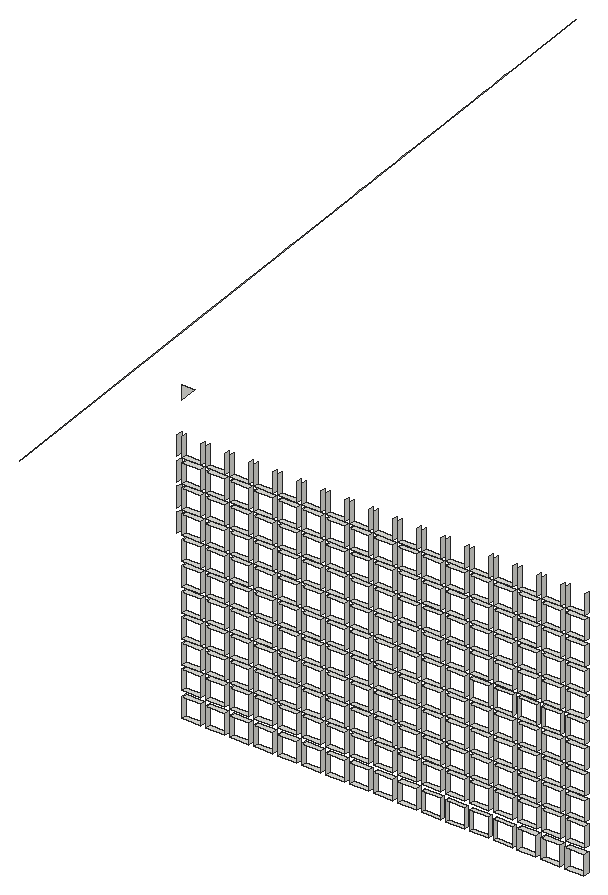
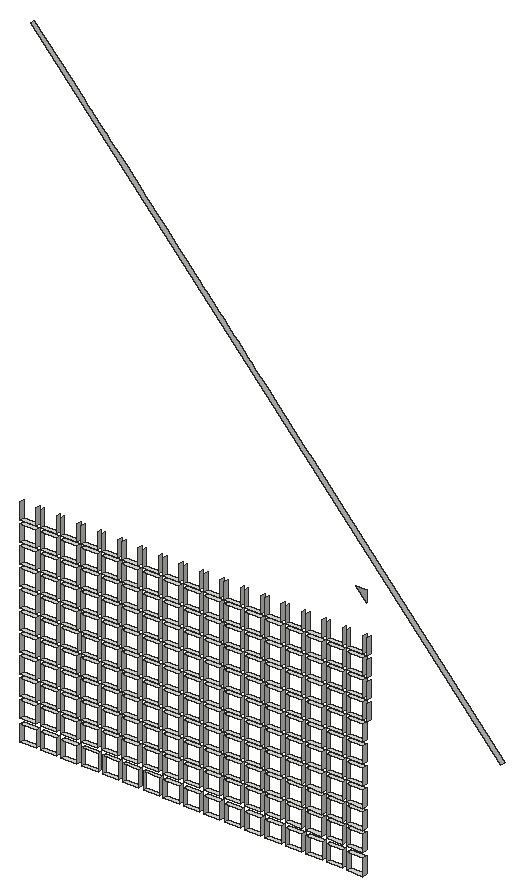
# SketchUp Ruby script. Lengths in inches.
U = 1.inch
M = Sketchup.active_model
def pt(a) = Geom::Point3d.new(a.map { |v| v * U })
def face(e, loops, mat)
  f = e.add_face(loops[0].map { |a| pt(a) })
  loops[1..].each { |l| e.add_face(l.map { |a| pt(a) }).erase! }
  f.material = f.back_material = mat if mat
  f
end
# faces: each face lists its corners as indices into pts; further lists are holes
def faces(e, pts, list, mat = nil) = list.each { |f| face(e, (f[0].is_a?(Array) ? f : [f]).map { |l| l.map { |i| pts[i] } }, mat) }
# xy, xz, yz: faces in a plane at the given z, y or x. An outline is a flat list of corners, or four numbers for a rectangle; further outlines are holes
def ring(l) = l.size == 4 ? [[l[0], l[1]], [l[2], l[1]], [l[2], l[3]], [l[0], l[3]]] : l.each_slice(2).to_a
def flat(e, list, mat, &to3) = list.each { |f| face(e, (f[0].is_a?(Array) ? f : [f]).map { |l| ring(l).map { |u, v| to3.(u, v) } }, mat) }
def xy(e, z, list, mat = nil) = flat(e, list, mat) { |x, y| [x, y, z] }
def xz(e, y, list, mat = nil) = flat(e, list, mat) { |x, z| [x, y, z] }
def yz(e, x, list, mat = nil) = flat(e, list, mat) { |y, z| [x, y, z] }
def lines(e, pts, list) = list.each { |a, b| e.add_line(pt(pts[a]), pt(pts[b])) }
# prism: a flat outline (further loops are holes) pulled along v
def prism(e, loops, v, mat = nil)
  f = face(e, loops, mat); d = Geom::Vector3d.new(v.map { |x| x * U })
  f.pushpull(f.normal.samedirection?(d) ? d.length : -d.length)
end
def box(e, o, s, mat = nil) = prism(e, [[o, [o[0] + s[0], o[1], o[2]], [o[0] + s[0], o[1] + s[1], o[2]], [o[0], o[1] + s[1], o[2]]]], [0, 0, s[2]], mat)
def at(x, y, z, deg = 0) = Geom::Transformation.translation(pt([x, y, z])) * Geom::Transformation.rotation(ORIGIN, Z_AXIS, deg.degrees)
def axes(o, x, y, z) = Geom::Transformation.new([*x, 0, *y, 0, *z, 0, *pt(o).to_a, 1])
def part(name) = M.definitions.add(name)
# library, detail: a bought-in or finely detailed component or shape, given as its bounding box
def library(name, o, s) = part(name).tap { |d| box(d.entities, o, s) }
def detail(e, o, s) = box(e.add_group.entities, o, s)
def put(e, d, t, mat = nil) = e.add_instance(d, t).tap { |i| i.material = mat if mat }
def group(e, t, mat = nil) = e.add_group.tap { |g| g.transformation = t; g.material = mat if mat }.entities
root = M.entities
xy(root,305.35,[[2223.57,480.14,2225.88,480.77],[2226.48,480.14,2228.79,480.77],[2229.39,480.14,2231.71,480.77],[2232.31,480.14,2234.62,480.77],[2235.22,480.14,2237.53,480.77],
  [2238.13,480.14,2240.44,480.77],[2241.04,480.14,2243.35,480.77],[2243.95,480.14,2246.27,480.77],[2246.87,480.14,2249.18,480.77],[2249.78,480.14,2252.09,480.77],
  [2252.6875,480.14,2255,480.64],[2255.6,480.14,2257.91,480.64],[2258.51,480.14,2260.83,480.64],[2261.43,480.14,2263.74,480.64],[2264.34,480.14,2266.65,480.77],
  [2267.25,480.14,2269.5625,480.77],[2270.16,480.14,2272.47,480.77]])
xy(root,307.67,[[2223.57,480.14,2225.88,480.77],[2226.48,480.14,2228.79,480.77],[2229.39,480.14,2231.71,480.77],[2232.31,480.14,2234.62,480.77],[2235.22,480.14,2237.53,480.77],
  [2238.13,480.14,2240.44,480.77],[2241.04,480.14,2243.35,480.77],[2243.95,480.14,2246.27,480.77],[2246.87,480.14,2249.18,480.77],[2249.78,480.14,2252.09,480.77],
  [2252.6875,480.14,2255,480.64],[2255.6,480.14,2257.91,480.64],[2258.51,480.14,2260.83,480.64],[2261.43,480.14,2263.74,480.64],[2264.34,480.14,2266.65,480.77],
  [2267.25,480.14,2269.5625,480.77],[2270.16,480.14,2272.47,480.77]])
xy(root,308.4,[[2223.6,480.14,2225.91,480.77],[2226.51,480.14,2228.82,480.77],[2229.42,480.14,2231.73,480.77],[2232.33,480.14,2234.65,480.77],[2235.25,480.14,2237.56,480.77],
  [2238.16,480.14,2240.47,480.77],[2241.07,480.14,2243.38,480.77],[2243.98,480.14,2246.29,480.77],[2246.89,480.14,2249.21,480.77],[2249.81,480.14,2252.12,480.77],
  [2252.72,480.14,2255.03,480.77],[2255.63,480.14,2257.94,480.77],[2258.54,480.14,2260.86,480.77],[2261.45,480.14,2263.77,480.77],[2264.37,480.14,2266.68,480.77],
  [2267.28,480.14,2269.59,480.77],[2270.19,480.14,2272.5,480.77]])
xy(root,310.71,[[2223.6,480.14,2225.91,480.77],[2226.51,480.14,2228.82,480.77],[2229.42,480.14,2231.73,480.77],[2232.33,480.14,2234.65,480.77],[2235.25,480.14,2237.56,480.77],
  [2238.16,480.14,2240.47,480.77],[2241.07,480.14,2243.38,480.77],[2243.98,480.14,2246.29,480.77],[2246.89,480.14,2249.21,480.77],[2249.81,480.14,2252.12,480.77],
  [2252.72,480.14,2255.03,480.77],[2255.63,480.14,2257.94,480.77],[2258.54,480.14,2260.86,480.77],[2261.45,480.14,2263.77,480.77],[2264.37,480.14,2266.68,480.77],
  [2267.28,480.14,2269.59,480.77],[2270.19,480.14,2272.5,480.77]])
xy(root,311.21,[[2223.6,480.14,2225.91,480.77],[2226.51,480.14,2228.82,480.77],[2229.42,480.14,2231.73,480.77],[2232.33,480.14,2234.65,480.77],[2235.25,480.14,2237.56,480.77],
  [2238.16,480.14,2240.47,480.77],[2241.07,480.14,2243.38,480.77],[2243.98,480.14,2246.29,480.77],[2246.89,480.14,2249.21,480.77],[2249.81,480.14,2252.12,480.77],
  [2252.72,480.14,2255.03,480.77],[2255.63,480.14,2257.94,480.77],[2258.54,480.14,2260.86,480.77],[2261.45,480.14,2263.77,480.77],[2264.37,480.14,2266.68,480.77],
  [2267.28,480.14,2269.59,480.77],[2270.19,480.14,2272.5,480.77]])
xy(root,313.52,[[2223.6,480.14,2225.91,480.77],[2226.51,480.14,2228.82,480.77],[2229.42,480.14,2231.73,480.77],[2232.33,480.14,2234.65,480.77],[2235.25,480.14,2237.56,480.77],
  [2238.16,480.14,2240.47,480.77],[2241.07,480.14,2243.38,480.77],[2243.98,480.14,2246.29,480.77],[2246.89,480.14,2249.21,480.77],[2249.81,480.14,2252.12,480.77],
  [2252.72,480.14,2255.03,480.77],[2255.63,480.14,2257.94,480.77],[2258.54,480.14,2260.86,480.77],[2261.45,480.14,2263.77,480.77],[2264.37,480.14,2266.68,480.77],
  [2267.28,480.14,2269.59,480.77],[2270.19,480.14,2272.5,480.77]])
xy(root,314.02,[[2223.6,480.14,2225.91,480.77],[2226.51,480.14,2228.82,480.77],[2229.42,480.14,2231.73,480.77],[2232.33,480.14,2234.65,480.77],[2235.25,480.14,2237.56,480.77],
  [2238.16,480.14,2240.47,480.77],[2241.07,480.14,2243.38,480.77],[2243.98,480.14,2246.29,480.77],[2246.89,480.14,2249.21,480.77],[2249.81,480.14,2252.12,480.77],
  [2252.72,480.14,2255.03,480.77],[2255.63,480.14,2257.94,480.77],[2258.54,480.14,2260.86,480.77],[2261.45,480.14,2263.77,480.77],[2264.37,480.14,2266.68,480.77],
  [2267.28,480.14,2269.59,480.77],[2270.19,480.14,2272.5,480.77]])
xy(root,316.34,[[2223.6,480.14,2225.91,480.77],[2226.51,480.14,2228.82,480.77],[2229.42,480.14,2231.73,480.77],[2232.33,480.14,2234.65,480.77],[2235.25,480.14,2237.56,480.77],
  [2238.16,480.14,2240.47,480.77],[2241.07,480.14,2243.38,480.77],[2243.98,480.14,2246.29,480.77],[2246.89,480.14,2249.21,480.77],[2249.81,480.14,2252.12,480.77],
  [2252.72,480.14,2255.03,480.77],[2255.63,480.14,2257.94,480.77],[2258.54,480.14,2260.86,480.77],[2261.45,480.14,2263.77,480.77],[2264.37,480.14,2266.68,480.77],
  [2267.28,480.14,2269.59,480.77],[2270.19,480.14,2272.5,480.77]])
xy(root,316.84,[[2223.6,480.14,2225.91,480.77],[2226.51,480.14,2228.82,480.77],[2229.42,480.14,2231.73,480.77],[2232.33,480.14,2234.65,480.77],[2235.25,480.14,2237.56,480.77],
  [2238.16,480.14,2240.47,480.77],[2241.07,480.14,2243.38,480.77],[2243.98,480.14,2246.29,480.77],[2246.89,480.14,2249.21,480.77],[2249.81,480.14,2252.12,480.77],
  [2252.72,480.14,2255.03,480.77],[2255.63,480.14,2257.94,480.77],[2258.54,480.14,2260.86,480.77],[2261.45,480.14,2263.77,480.77],[2264.37,480.14,2266.68,480.77],
  [2267.28,480.14,2269.59,480.77],[2270.19,480.14,2272.5,480.77]])
xy(root,319.15,[[2223.6,480.14,2225.91,480.77],[2226.51,480.14,2228.82,480.77],[2229.42,480.14,2231.73,480.77],[2232.33,480.14,2234.65,480.77],[2235.25,480.14,2237.56,480.77],
  [2238.16,480.14,2240.47,480.77],[2241.07,480.14,2243.38,480.77],[2243.98,480.14,2246.29,480.77],[2246.89,480.14,2249.21,480.77],[2249.81,480.14,2252.12,480.77],
  [2252.72,480.14,2255.03,480.77],[2255.63,480.14,2257.94,480.77],[2258.54,480.14,2260.86,480.77],[2261.45,480.14,2263.77,480.77],[2264.37,480.14,2266.68,480.77],
  [2267.28,480.14,2269.59,480.77],[2270.19,480.14,2272.5,480.77]])
xy(root,319.65,[[2223.6,480.14,2225.91,480.77],[2226.51,480.14,2228.82,480.77],[2229.42,480.14,2231.73,480.77],[2232.33,480.14,2234.65,480.77],[2235.25,480.14,2237.56,480.77],
  [2238.16,480.14,2240.47,480.77],[2241.07,480.14,2243.38,480.77],[2243.98,480.14,2246.29,480.77],[2246.89,480.14,2249.21,480.77],[2249.81,480.14,2252.12,480.77],
  [2252.72,480.14,2255.03,480.77],[2255.63,480.14,2257.94,480.77],[2258.54,480.14,2260.86,480.7],[2261.45,480.14,2263.77,480.7],[2264.37,480.14,2266.68,480.7],
  [2267.28,480.14,2269.59,480.7],[2270.19,480.14,2272.5,480.77]])
xy(root,321.96,[[2223.6,480.14,2225.91,480.77],[2226.51,480.14,2228.82,480.77],[2229.42,480.14,2231.73,480.77],[2232.33,480.14,2234.65,480.77],[2235.25,480.14,2237.56,480.77],
  [2238.16,480.14,2240.47,480.77],[2241.07,480.14,2243.38,480.77],[2243.98,480.14,2246.29,480.77],[2246.89,480.14,2249.21,480.77],[2249.81,480.14,2252.12,480.77],
  [2252.72,480.14,2255.03,480.77],[2255.63,480.14,2257.94,480.77],[2258.54,480.14,2260.86,480.7],[2261.45,480.14,2263.77,480.7],[2264.37,480.14,2266.68,480.7],
  [2267.28,480.14,2269.59,480.7],[2270.19,480.14,2272.5,480.77]])
xy(root,322.46,[[2223.6,480.14,2225.91,480.77],[2226.51,480.14,2228.82,480.77],[2229.42,480.14,2231.73,480.77],[2232.33,480.14,2234.65,480.77],[2235.25,480.14,2237.56,480.77],
  [2238.16,480.14,2240.47,480.77],[2241.07,480.14,2243.38,480.77],[2243.98,480.14,2246.29,480.77],[2246.89,480.14,2249.21,480.77],[2249.81,480.14,2252.12,480.77],
  [2252.72,480.14,2255.03,480.77],[2255.63,480.14,2257.94,480.77],[2258.54,480.14,2260.86,480.77],[2261.45,480.14,2263.77,480.77],[2264.37,480.14,2266.68,480.77],
  [2267.28,480.14,2269.59,480.77],[2270.19,480.14,2272.5,480.77]])
xy(root,324.77,[[2223.6,480.14,2225.91,480.77],[2226.51,480.14,2228.82,480.77],[2229.42,480.14,2231.73,480.77],[2232.33,480.14,2234.65,480.77],[2235.25,480.14,2237.56,480.77],
  [2238.16,480.14,2240.47,480.77],[2241.07,480.14,2243.38,480.77],[2243.98,480.14,2246.29,480.77],[2246.89,480.14,2249.21,480.77],[2249.81,480.14,2252.12,480.77],
  [2252.72,480.14,2255.03,480.77],[2255.63,480.14,2257.94,480.77],[2258.54,480.14,2260.86,480.77],[2261.45,480.14,2263.77,480.77],[2264.37,480.14,2266.68,480.77],
  [2267.28,480.14,2269.59,480.77],[2270.19,480.14,2272.5,480.77]])
xy(root,325.27,[[2223.6,480.14,2225.91,480.77],[2226.51,480.14,2228.82,480.77],[2229.42,480.14,2231.73,480.77],[2232.33,480.14,2234.65,480.77],[2235.25,480.14,2237.56,480.77],
  [2238.16,480.14,2240.47,480.77],[2241.07,480.14,2243.38,480.77],[2243.98,480.14,2246.29,480.77],[2246.89,480.14,2249.21,480.77],[2249.81,480.14,2252.12,480.77],
  [2252.72,480.14,2255.03,480.77],[2255.63,480.14,2257.94,480.77],[2258.54,480.14,2260.86,480.77],[2261.45,480.14,2263.77,480.77],[2264.37,480.14,2266.68,480.77],
  [2267.28,480.14,2269.59,480.77],[2270.19,480.14,2272.5,480.77]])
xy(root,327.59,[[2223.6,480.14,2225.91,480.77],[2226.51,480.14,2228.82,480.77],[2229.42,480.14,2231.73,480.77],[2232.33,480.14,2234.65,480.77],[2235.25,480.14,2237.56,480.77],
  [2238.16,480.14,2240.47,480.77],[2241.07,480.14,2243.38,480.77],[2243.98,480.14,2246.29,480.77],[2246.89,480.14,2249.21,480.77],[2249.81,480.14,2252.12,480.77],
  [2252.72,480.14,2255.03,480.77],[2255.63,480.14,2257.94,480.77],[2258.54,480.14,2260.86,480.77],[2261.45,480.14,2263.77,480.77],[2264.37,480.14,2266.68,480.77],
  [2267.28,480.14,2269.59,480.77],[2270.19,480.14,2272.5,480.77]])
xy(root,328.09,[[2223.6,480.14,2225.91,480.77],[2226.51,480.14,2228.82,480.77],[2229.42,480.14,2231.73,480.77],[2232.33,480.14,2234.65,480.77],[2235.25,480.14,2237.56,480.77],
  [2238.16,480.14,2240.47,480.77],[2241.07,480.14,2243.38,480.77],[2243.98,480.14,2246.29,480.77],[2246.89,480.14,2249.21,480.77],[2249.81,480.14,2252.12,480.77],
  [2252.72,480.14,2255.03,480.77],[2255.63,480.14,2257.94,480.77],[2258.54,480.14,2260.86,480.77],[2261.45,480.14,2263.77,480.77],[2264.37,480.14,2266.68,480.77],
  [2267.28,480.14,2269.59,480.77],[2270.19,480.14,2272.5,480.77]])
xy(root,330.4,[[2223.6,480.14,2225.91,480.77],[2226.51,480.14,2228.82,480.77],[2229.42,480.14,2231.73,480.77],[2232.33,480.14,2234.65,480.77],[2235.25,480.14,2237.56,480.77],
  [2238.16,480.14,2240.47,480.77],[2241.07,480.14,2243.38,480.77],[2243.98,480.14,2246.29,480.77],[2246.89,480.14,2249.21,480.77],[2249.81,480.14,2252.12,480.77],
  [2252.72,480.14,2255.03,480.77],[2255.63,480.14,2257.94,480.77],[2258.54,480.14,2260.86,480.77],[2261.45,480.14,2263.77,480.77],[2264.37,480.14,2266.68,480.77],
  [2267.28,480.14,2269.59,480.77],[2270.19,480.14,2272.5,480.77]])
xy(root,330.9,[[2223.6,480.14,2225.91,480.77],[2226.51,480.14,2228.82,480.77],[2229.42,480.14,2231.73,480.77],[2232.33,480.14,2234.65,480.77],[2235.25,480.14,2237.56,480.77],
  [2238.16,480.14,2240.47,480.77],[2241.07,480.14,2243.38,480.77],[2243.98,480.14,2246.29,480.77],[2246.89,480.14,2249.21,480.77],[2249.81,480.14,2252.12,480.77],
  [2252.72,480.14,2255.03,480.77],[2255.63,480.14,2257.94,480.77],[2258.54,480.14,2260.86,480.77],[2261.45,480.14,2263.77,480.77],[2264.37,480.14,2266.68,480.77],
  [2267.28,480.14,2269.59,480.77],[2270.19,480.14,2272.5,480.77]])
xy(root,333.21,[[2223.6,480.14,2225.91,480.77],[2226.51,480.14,2228.82,480.77],[2229.42,480.14,2231.73,480.77],[2232.33,480.14,2234.65,480.77],[2235.25,480.14,2237.56,480.77],
  [2238.16,480.14,2240.47,480.77],[2241.07,480.14,2243.38,480.77],[2243.98,480.14,2246.29,480.77],[2246.89,480.14,2249.21,480.77],[2249.81,480.14,2252.12,480.77],
  [2252.72,480.14,2255.03,480.77],[2255.63,480.14,2257.94,480.77],[2258.54,480.14,2260.86,480.77],[2261.45,480.14,2263.77,480.77],[2264.37,480.14,2266.68,480.77],
  [2267.28,480.14,2269.59,480.77],[2270.19,480.14,2272.5,480.77]])
xy(root,333.71,[[2223.6,480.14,2225.91,480.77],[2226.51,480.14,2228.82,480.77],[2229.42,480.14,2231.73,480.77],[2232.33,480.14,2234.65,480.77],[2235.25,480.14,2237.56,480.77],
  [2238.16,480.14,2240.47,480.77],[2241.07,480.14,2243.38,480.77],[2243.98,480.14,2246.29,480.77],[2246.89,480.14,2249.21,480.77],[2249.81,480.14,2252.12,480.77],
  [2252.72,480.14,2255.03,480.77],[2255.63,480.14,2257.94,480.77],[2258.54,480.14,2260.86,480.77],[2261.45,480.14,2263.77,480.77],[2264.37,480.14,2266.68,480.77],
  [2267.28,480.14,2269.59,480.77],[2270.19,480.14,2272.5,480.77]])
xz(root,480.14,[[2223.6,340.04,2225.11,341.65,2223.6,341.65]])
yz(root,2223,[[480.14,325.27,480.77,327.59],[480.14,328.09,480.77,330.4],[480.14,330.9,480.77,333.21],[480.14,333.71,480.77,336.02]])
yz(root,2223.57,[[480.14,305.35,480.77,307.67]])
yz(root,2223.6,[[480.14,308.4,480.77,310.71],[480.14,311.21,480.77,313.52],[480.14,314.02,480.77,316.34],[480.14,316.84,480.77,319.15],[480.14,319.65,480.77,321.96],
  [480.14,322.46,480.77,324.77],[480.14,325.27,480.77,327.59],[480.14,328.09,480.77,330.4],[480.14,330.9,480.77,333.21],[480.14,333.71,480.77,336.02]])
yz(root,2225.88,[[480.14,305.35,480.77,307.67]])
yz(root,2225.91,[[480.14,308.4,480.77,310.71],[480.14,311.21,480.77,313.52],[480.14,314.02,480.77,316.34],[480.14,316.84,480.77,319.15],[480.14,319.65,480.77,321.96],
  [480.14,322.46,480.77,324.77],[480.14,325.27,480.77,327.59],[480.14,328.09,480.77,330.4],[480.14,330.9,480.77,333.21],[480.14,333.71,480.77,336.02]])
yz(root,2226.48,[[480.14,305.35,480.77,307.67]])
yz(root,2226.51,[[480.14,308.4,480.77,310.71],[480.14,311.21,480.77,313.52],[480.14,314.02,480.77,316.34],[480.14,316.84,480.77,319.15],[480.14,319.65,480.77,321.96],
  [480.14,322.46,480.77,324.77],[480.14,325.27,480.77,327.59],[480.14,328.09,480.77,330.4],[480.14,330.9,480.77,333.21],[480.14,333.71,480.77,336.02]])
yz(root,2228.79,[[480.14,305.35,480.77,307.67]])
yz(root,2228.82,[[480.14,308.4,480.77,310.71],[480.14,311.21,480.77,313.52],[480.14,314.02,480.77,316.34],[480.14,316.84,480.77,319.15],[480.14,319.65,480.77,321.96],
  [480.14,322.46,480.77,324.77],[480.14,325.27,480.77,327.59],[480.14,328.09,480.77,330.4],[480.14,330.9,480.77,333.21],[480.14,333.71,480.77,336.02]])
yz(root,2229.39,[[480.14,305.35,480.77,307.67]])
yz(root,2229.42,[[480.14,308.4,480.77,310.71],[480.14,311.21,480.77,313.52],[480.14,314.02,480.77,316.34],[480.14,316.84,480.77,319.15],[480.14,319.65,480.77,321.96],
  [480.14,322.46,480.77,324.77],[480.14,325.27,480.77,327.59],[480.14,328.09,480.77,330.4],[480.14,330.9,480.77,333.21],[480.14,333.71,480.77,336.02]])
yz(root,2231.71,[[480.14,305.35,480.77,307.67]])
yz(root,2231.73,[[480.14,308.4,480.77,310.71],[480.14,311.21,480.77,313.52],[480.14,314.02,480.77,316.34],[480.14,316.84,480.77,319.15],[480.14,319.65,480.77,321.96],
  [480.14,322.46,480.77,324.77],[480.14,325.27,480.77,327.59],[480.14,328.09,480.77,330.4],[480.14,330.9,480.77,333.21],[480.14,333.71,480.77,336.02]])
yz(root,2232.31,[[480.14,305.35,480.77,307.67]])
yz(root,2232.33,[[480.14,308.4,480.77,310.71],[480.14,311.21,480.77,313.52],[480.14,314.02,480.77,316.34],[480.14,316.84,480.77,319.15],[480.14,319.65,480.77,321.96],
  [480.14,322.46,480.77,324.77],[480.14,325.27,480.77,327.59],[480.14,328.09,480.77,330.4],[480.14,330.9,480.77,333.21],[480.14,333.71,480.77,336.02]])
yz(root,2234.62,[[480.14,305.35,480.77,307.67]])
yz(root,2234.65,[[480.14,308.4,480.77,310.71],[480.14,311.21,480.77,313.52],[480.14,314.02,480.77,316.34],[480.14,316.84,480.77,319.15],[480.14,319.65,480.77,321.96],
  [480.14,322.46,480.77,324.77],[480.14,325.27,480.77,327.59],[480.14,328.09,480.77,330.4],[480.14,330.9,480.77,333.21],[480.14,333.71,480.77,336.02]])
yz(root,2235.22,[[480.14,305.35,480.77,307.67]])
yz(root,2235.25,[[480.14,308.4,480.77,310.71],[480.14,311.21,480.77,313.52],[480.14,314.02,480.77,316.34],[480.14,316.84,480.77,319.15],[480.14,319.65,480.77,321.96],
  [480.14,322.46,480.77,324.77],[480.14,325.27,480.77,327.59],[480.14,328.09,480.77,330.4],[480.14,330.9,480.77,333.21],[480.14,333.71,480.77,336.02]])
yz(root,2237.53,[[480.14,305.35,480.77,307.67]])
yz(root,2237.56,[[480.14,308.4,480.77,310.71],[480.14,311.21,480.77,313.52],[480.14,314.02,480.77,316.34],[480.14,316.84,480.77,319.15],[480.14,319.65,480.77,321.96],
  [480.14,322.46,480.77,324.77],[480.14,325.27,480.77,327.59],[480.14,328.09,480.77,330.4],[480.14,330.9,480.77,333.21],[480.14,333.71,480.77,336.02]])
yz(root,2238.13,[[480.14,305.35,480.77,307.67]])
yz(root,2238.16,[[480.14,308.4,480.77,310.71],[480.14,311.21,480.77,313.52],[480.14,314.02,480.77,316.34],[480.14,316.84,480.77,319.15],[480.14,319.65,480.77,321.96],
  [480.14,322.46,480.77,324.77],[480.14,325.27,480.77,327.59],[480.14,328.09,480.77,330.4],[480.14,330.9,480.77,333.21],[480.14,333.71,480.77,336.02]])
yz(root,2240.44,[[480.14,305.35,480.77,307.67]])
yz(root,2240.47,[[480.14,308.4,480.77,310.71],[480.14,311.21,480.77,313.52],[480.14,314.02,480.77,316.34],[480.14,316.84,480.77,319.15],[480.14,319.65,480.77,321.96],
  [480.14,322.46,480.77,324.77],[480.14,325.27,480.77,327.59],[480.14,328.09,480.77,330.4],[480.14,330.9,480.77,333.21],[480.14,333.71,480.77,336.02]])
yz(root,2241.04,[[480.14,305.35,480.77,307.67]])
yz(root,2241.07,[[480.14,308.4,480.77,310.71],[480.14,311.21,480.77,313.52],[480.14,314.02,480.77,316.34],[480.14,316.84,480.77,319.15],[480.14,319.65,480.77,321.96],
  [480.14,322.46,480.77,324.77],[480.14,325.27,480.77,327.59],[480.14,328.09,480.77,330.4],[480.14,330.9,480.77,333.21],[480.14,333.71,480.77,336.02]])
yz(root,2243.35,[[480.14,305.35,480.77,307.67]])
yz(root,2243.38,[[480.14,308.4,480.77,310.71],[480.14,311.21,480.77,313.52],[480.14,314.02,480.77,316.34],[480.14,316.84,480.77,319.15],[480.14,319.65,480.77,321.96],
  [480.14,322.46,480.77,324.77],[480.14,325.27,480.77,327.59],[480.14,328.09,480.77,330.4],[480.14,330.9,480.77,333.21],[480.14,333.71,480.77,336.02]])
yz(root,2243.95,[[480.14,305.35,480.77,307.67]])
yz(root,2243.98,[[480.14,308.4,480.77,310.71],[480.14,311.21,480.77,313.52],[480.14,314.02,480.77,316.34],[480.14,316.84,480.77,319.15],[480.14,319.65,480.77,321.96],
  [480.14,322.46,480.77,324.77],[480.14,325.27,480.77,327.59],[480.14,328.09,480.77,330.4],[480.14,330.9,480.77,333.21],[480.14,333.71,480.77,336.02]])
yz(root,2246.27,[[480.14,305.35,480.77,307.67]])
yz(root,2246.29,[[480.14,308.4,480.77,310.71],[480.14,311.21,480.77,313.52],[480.14,314.02,480.77,316.34],[480.14,316.84,480.77,319.15],[480.14,319.65,480.77,321.96],
  [480.14,322.46,480.77,324.77],[480.14,325.27,480.77,327.59],[480.14,328.09,480.77,330.4],[480.14,330.9,480.77,333.21],[480.14,333.71,480.77,336.02]])
yz(root,2246.87,[[480.14,305.35,480.77,307.67]])
yz(root,2246.89,[[480.14,308.4,480.77,310.71],[480.14,311.21,480.77,313.52],[480.14,314.02,480.77,316.34],[480.14,316.84,480.77,319.15],[480.14,319.65,480.77,321.96],
  [480.14,322.46,480.77,324.77],[480.14,325.27,480.77,327.59],[480.14,328.09,480.77,330.4],[480.14,330.9,480.77,333.21],[480.14,333.71,480.77,336.02]])
yz(root,2249.18,[[480.14,305.35,480.77,307.67]])
yz(root,2249.21,[[480.14,308.4,480.77,310.71],[480.14,311.21,480.77,313.52],[480.14,314.02,480.77,316.34],[480.14,316.84,480.77,319.15],[480.14,319.65,480.77,321.96],
  [480.14,322.46,480.77,324.77],[480.14,325.27,480.77,327.59],[480.14,328.09,480.77,330.4],[480.14,330.9,480.77,333.21],[480.14,333.71,480.77,336.02]])
yz(root,2249.78,[[480.14,305.35,480.77,307.67]])
yz(root,2249.81,[[480.14,308.4,480.77,310.71],[480.14,311.21,480.77,313.52],[480.14,314.02,480.77,316.34],[480.14,316.84,480.77,319.15],[480.14,319.65,480.77,321.96],
  [480.14,322.46,480.77,324.77],[480.14,325.27,480.77,327.59],[480.14,328.09,480.77,330.4],[480.14,330.9,480.77,333.21],[480.14,333.71,480.77,336.02]])
yz(root,2252.09,[[480.14,305.35,480.77,307.67]])
yz(root,2252.12,[[480.14,308.4,480.77,310.71],[480.14,311.21,480.77,313.52],[480.14,314.02,480.77,316.34],[480.14,316.84,480.77,319.15],[480.14,319.65,480.77,321.96],
  [480.14,322.46,480.77,324.77],[480.14,325.27,480.77,327.59],[480.14,328.09,480.77,330.4],[480.14,330.9,480.77,333.21],[480.14,333.71,480.77,336.02]])
yz(root,2252.6875,[[480.14,305.35,480.64,307.67]])
yz(root,2252.72,[[480.14,308.4,480.77,310.71],[480.14,311.21,480.77,313.52],[480.14,314.02,480.77,316.34],[480.14,316.84,480.77,319.15],[480.14,319.65,480.77,321.96],
  [480.14,322.46,480.77,324.77],[480.14,325.27,480.77,327.59],[480.14,328.09,480.77,330.4],[480.14,330.9,480.77,333.21],[480.14,333.71,480.77,336.02]])
yz(root,2255,[[480.14,305.35,480.64,307.67]])
yz(root,2255.03,[[480.14,308.4,480.77,310.71],[480.14,311.21,480.77,313.52],[480.14,314.02,480.77,316.34],[480.14,316.84,480.77,319.15],[480.14,319.65,480.77,321.96],
  [480.14,322.46,480.77,324.77],[480.14,325.27,480.77,327.59],[480.14,328.09,480.77,330.4],[480.14,330.9,480.77,333.21],[480.14,333.71,480.77,336.02]])
yz(root,2255.6,[[480.14,305.35,480.64,307.67]])
yz(root,2255.63,[[480.14,308.4,480.77,310.71],[480.14,311.21,480.77,313.52],[480.14,314.02,480.77,316.34],[480.14,316.84,480.77,319.15],[480.14,319.65,480.77,321.96],
  [480.14,322.46,480.77,324.77],[480.14,325.27,480.77,327.59],[480.14,328.09,480.77,330.4],[480.14,330.9,480.77,333.21],[480.14,333.71,480.77,336.02]])
yz(root,2257.91,[[480.14,305.35,480.64,307.67]])
yz(root,2257.94,[[480.14,308.4,480.77,310.71],[480.14,311.21,480.77,313.52],[480.14,314.02,480.77,316.34],[480.14,316.84,480.77,319.15],[480.14,319.65,480.77,321.96],
  [480.14,322.46,480.77,324.77],[480.14,325.27,480.77,327.59],[480.14,328.09,480.77,330.4],[480.14,330.9,480.77,333.21],[480.14,333.71,480.77,336.02]])
yz(root,2258.51,[[480.14,305.35,480.64,307.67]])
yz(root,2258.54,[[480.14,308.4,480.77,310.71],[480.14,311.21,480.77,313.52],[480.14,314.02,480.77,316.34],[480.14,316.84,480.77,319.15],[480.14,319.65,480.7,321.96],
  [480.14,322.46,480.77,324.77],[480.14,325.27,480.77,327.59],[480.14,328.09,480.77,330.4],[480.14,330.9,480.77,333.21],[480.14,333.71,480.77,336.02]])
yz(root,2260.83,[[480.14,305.35,480.64,307.67]])
yz(root,2260.86,[[480.14,308.4,480.77,310.71],[480.14,311.21,480.77,313.52],[480.14,314.02,480.77,316.34],[480.14,316.84,480.77,319.15],[480.14,319.65,480.7,321.96],
  [480.14,322.46,480.77,324.77],[480.14,325.27,480.77,327.59],[480.14,328.09,480.77,330.4],[480.14,330.9,480.77,333.21],[480.14,333.71,480.77,336.02]])
yz(root,2261.43,[[480.14,305.35,480.64,307.67]])
yz(root,2261.45,[[480.14,308.4,480.77,310.71],[480.14,311.21,480.77,313.52],[480.14,314.02,480.77,316.34],[480.14,316.84,480.77,319.15],[480.14,319.65,480.7,321.96],
  [480.14,322.46,480.77,324.77],[480.14,325.27,480.77,327.59],[480.14,328.09,480.77,330.4],[480.14,330.9,480.77,333.21],[480.14,333.71,480.77,336.02]])
yz(root,2263.74,[[480.14,305.35,480.64,307.67]])
yz(root,2263.77,[[480.14,308.4,480.77,310.71],[480.14,311.21,480.77,313.52],[480.14,314.02,480.77,316.34],[480.14,316.84,480.77,319.15],[480.14,319.65,480.7,321.96],
  [480.14,322.46,480.77,324.77],[480.14,325.27,480.77,327.59],[480.14,328.09,480.77,330.4],[480.14,330.9,480.77,333.21],[480.14,333.71,480.77,336.02]])
yz(root,2264.34,[[480.14,305.35,480.77,307.67]])
yz(root,2264.37,[[480.14,308.4,480.77,310.71],[480.14,311.21,480.77,313.52],[480.14,314.02,480.77,316.34],[480.14,316.84,480.77,319.15],[480.14,319.65,480.7,321.96],
  [480.14,322.46,480.77,324.77],[480.14,325.27,480.77,327.59],[480.14,328.09,480.77,330.4],[480.14,330.9,480.77,333.21],[480.14,333.71,480.77,336.02]])
yz(root,2266.65,[[480.14,305.35,480.77,307.67]])
yz(root,2266.68,[[480.14,308.4,480.77,310.71],[480.14,311.21,480.77,313.52],[480.14,314.02,480.77,316.34],[480.14,316.84,480.77,319.15],[480.14,319.65,480.7,321.96],
  [480.14,322.46,480.77,324.77],[480.14,325.27,480.77,327.59],[480.14,328.09,480.77,330.4],[480.14,330.9,480.77,333.21],[480.14,333.71,480.77,336.02]])
yz(root,2267.25,[[480.14,305.35,480.77,307.67]])
yz(root,2267.28,[[480.14,308.4,480.77,310.71],[480.14,311.21,480.77,313.52],[480.14,314.02,480.77,316.34],[480.14,316.84,480.77,319.15],[480.14,319.65,480.7,321.96],
  [480.14,322.46,480.77,324.77],[480.14,325.27,480.77,327.59],[480.14,328.09,480.77,330.4],[480.14,330.9,480.77,333.21],[480.14,333.71,480.77,336.02]])
yz(root,2269.5625,[[480.14,305.35,480.77,307.67]])
yz(root,2269.59,[[480.14,308.4,480.77,310.71],[480.14,311.21,480.77,313.52],[480.14,314.02,480.77,316.34],[480.14,316.84,480.77,319.15],[480.14,319.65,480.7,321.96],
  [480.14,322.46,480.77,324.77],[480.14,325.27,480.77,327.59],[480.14,328.09,480.77,330.4],[480.14,330.9,480.77,333.21],[480.14,333.71,480.77,336.02]])
yz(root,2270.16,[[480.14,305.35,480.77,307.67]])
yz(root,2270.19,[[480.14,308.4,480.77,310.71],[480.14,311.21,480.77,313.52],[480.14,314.02,480.77,316.34],[480.14,316.84,480.77,319.15],[480.14,319.65,480.77,321.96],
  [480.14,322.46,480.77,324.77],[480.14,325.27,480.77,327.59],[480.14,328.09,480.77,330.4],[480.14,330.9,480.77,333.21],[480.14,333.71,480.77,336.02]])
yz(root,2272.47,[[480.14,305.35,480.77,307.67]])
yz(root,2272.5,[[480.14,308.4,480.77,310.71],[480.14,311.21,480.77,313.52],[480.14,314.02,480.77,316.34],[480.14,316.84,480.77,319.15],[480.14,319.65,480.77,321.96],
  [480.14,322.46,480.77,324.77],[480.14,325.27,480.77,327.59],[480.14,328.09,480.77,330.4],[480.14,330.9,480.77,333.21],[480.14,333.71,480.77,336.02]])
p = [[2265.46,480.14,391.9],[2270.96,480.14,397.75],[2270.96,480.77,397.75],[2203.9,480.77,326.5],[2203.9,480.14,326.5],[2226.57,480.14,350.59],
  [2228.75,480.14,352.9],[2229.42,480.14,353.62],[2231.4,480.14,355.71],[2232.33,480.14,356.71],[2234.04,480.14,358.52],[2234.51,480.14,359.02],
  [2234.65,480.14,359.17],[2235.25,480.14,359.8],[2236.69,480.14,361.34],[2237.16,480.14,361.84],[2237.56,480.14,362.26],[2238.16,480.14,362.9],
  [2239.34,480.14,364.15],[2239.81,480.14,364.65],[2240.47,480.14,365.35],[2241.07,480.14,365.99],[2241.99,480.14,366.96],[2242.46,480.14,367.46],
  [2243.38,480.14,368.45],[2243.98,480.14,369.08],[2244.63,480.14,369.77],[2245.1,480.14,370.27],[2246.29,480.14,371.54],[2246.89,480.14,372.18],
  [2247.28,480.14,372.59],[2247.75,480.14,373.09],[2249.21,480.14,374.63],[2249.81,480.14,375.27],[2249.93,480.14,375.4],[2250.34,480.14,375.84],
  [2252.12,480.14,377.73],[2252.93,480.14,378.59],[2255.03,480.14,380.82],[2255.63,480.14,381.46],[2257.69,480.14,383.65],[2258.54,480.14,384.55],
  [2260.28,480.14,386.4],[2260.69,480.14,386.84],[2260.86,480.14,387.01],[2261.45,480.14,387.65],[2262.87,480.14,389.15],[2263.28,480.14,389.59],
  [2263.77,480.14,390.1],[2264.37,480.14,390.74]]
faces(root,p,[[0,1,2,3,4,5,6,7,8,9,10,11,12,13,14,15,16,17,18,19,20,21,22,23,24,25,26,27,28,29,30,31,32,33,34,35,36,37,38,39,40,41,42,43,44,45,46,47,48,49]])
